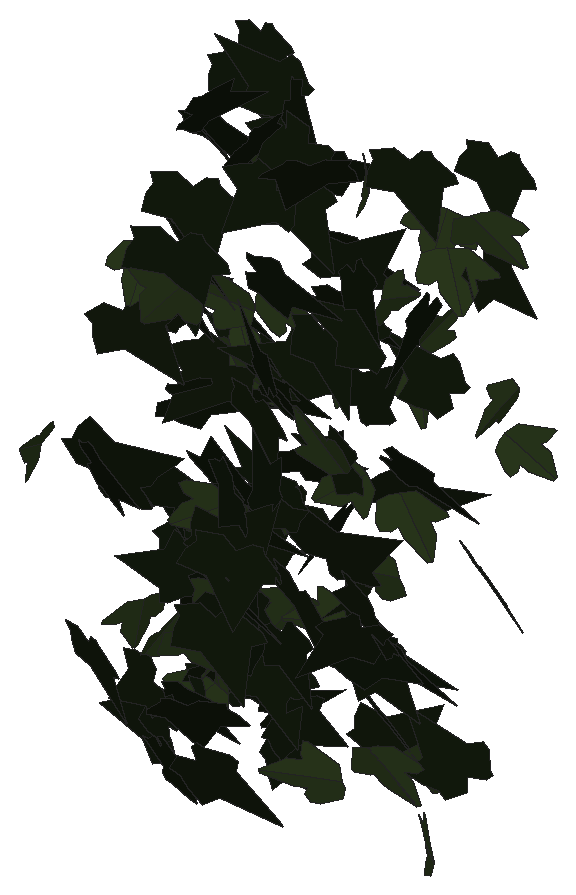
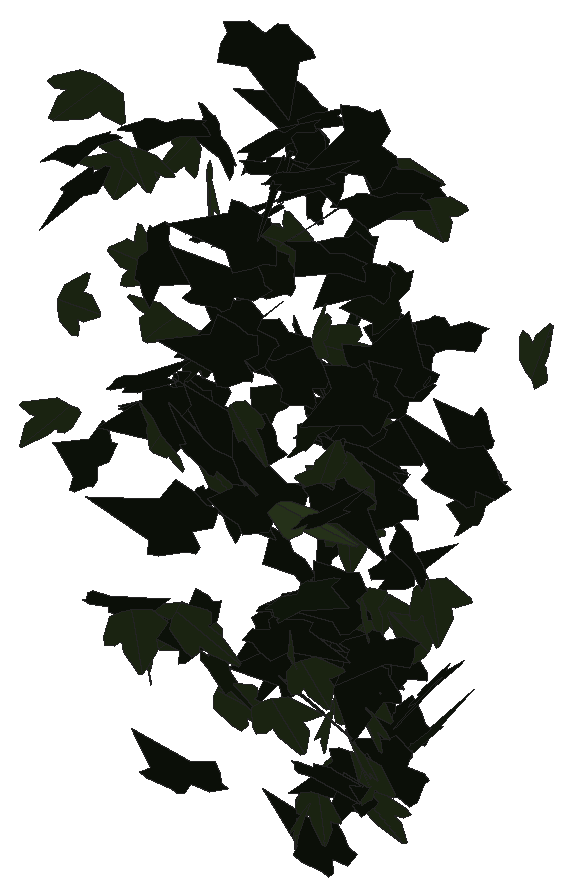
# SketchUp Ruby script. Lengths in inches.
U = 1.inch
M = Sketchup.active_model
def pt(a) = Geom::Point3d.new(a.map { |v| v * U })
def face(e, loops, mat)
  f = e.add_face(loops[0].map { |a| pt(a) })
  loops[1..].each { |l| e.add_face(l.map { |a| pt(a) }).erase! }
  f.material = f.back_material = mat if mat
  f
end
# faces: each face lists its corners as indices into pts; further lists are holes
def faces(e, pts, list, mat = nil) = list.each { |f| face(e, (f[0].is_a?(Array) ? f : [f]).map { |l| l.map { |i| pts[i] } }, mat) }
# xy, xz, yz: faces in a plane at the given z, y or x. An outline is a flat list of corners, or four numbers for a rectangle; further outlines are holes
def ring(l) = l.size == 4 ? [[l[0], l[1]], [l[2], l[1]], [l[2], l[3]], [l[0], l[3]]] : l.each_slice(2).to_a
def flat(e, list, mat, &to3) = list.each { |f| face(e, (f[0].is_a?(Array) ? f : [f]).map { |l| ring(l).map { |u, v| to3.(u, v) } }, mat) }
def xy(e, z, list, mat = nil) = flat(e, list, mat) { |x, y| [x, y, z] }
def xz(e, y, list, mat = nil) = flat(e, list, mat) { |x, z| [x, y, z] }
def yz(e, x, list, mat = nil) = flat(e, list, mat) { |y, z| [x, y, z] }
def lines(e, pts, list) = list.each { |a, b| e.add_line(pt(pts[a]), pt(pts[b])) }
# prism: a flat outline (further loops are holes) pulled along v
def prism(e, loops, v, mat = nil)
  f = face(e, loops, mat); d = Geom::Vector3d.new(v.map { |x| x * U })
  f.pushpull(f.normal.samedirection?(d) ? d.length : -d.length)
end
def box(e, o, s, mat = nil) = prism(e, [[o, [o[0] + s[0], o[1], o[2]], [o[0] + s[0], o[1] + s[1], o[2]], [o[0], o[1] + s[1], o[2]]]], [0, 0, s[2]], mat)
def at(x, y, z, deg = 0) = Geom::Transformation.translation(pt([x, y, z])) * Geom::Transformation.rotation(ORIGIN, Z_AXIS, deg.degrees)
def axes(o, x, y, z) = Geom::Transformation.new([*x, 0, *y, 0, *z, 0, *pt(o).to_a, 1])
def part(name) = M.definitions.add(name)
# library, detail: a bought-in or finely detailed component or shape, given as its bounding box
def library(name, o, s) = part(name).tap { |d| box(d.entities, o, s) }
def detail(e, o, s) = box(e.add_group.entities, o, s)
def put(e, d, t, mat = nil) = e.add_instance(d, t).tap { |i| i.material = mat if mat }
def group(e, t, mat = nil) = e.add_group.tap { |g| g.transformation = t; g.material = mat if mat }.entities
root = M.entities
M.materials.add("1026 AP 7946 SUNNY SIDE UP").color = [254, 231, 186]
M.materials.add("efeu1").color = [18, 25, 13]
M.materials.add("efeu2").color = [43, 57, 29]
c1 = part("ivyleaf_10")
p = [[0,0.5,-0.03],[-0.0625,2.02,-0.43],[-0.19,2.01,-0.46],[-0.54,1.05,-0.29],[-0.52,0.625,-0.18],[-0.83,0.76,-0.28],
  [-1.16,0.64,-0.33],[-1.15,0.33,-0.24],[-0.77,-0.39,0.02],[-0.3,-0.51,0.16],[0.04,-0.48,0.23],[-0.02,2.01,-0.4375],
  [-0.06,2.01,-0.43],[0.04,-0.49,0.23],[0.67,-0.49,0.14],[1.38,0.36,-0.2],[1.375,0.51,-0.24],[0.81,0.65,-0.19],
  [0.62,0.59,-0.15],[0.6,1.09,-0.28],[0.5,1.23,-0.31]]
faces(c1.entities,p,[[0,1,2,3,4,5,6,7,8,9,10],[11,12,0,13,14,15,16,17,18,19,20]],"efeu2")
c2 = part("ivyleaf_9")
p = [[1.54,2.16,1.25],[1.36,2.04,1.19],[-0.21,0.99,0.68],[-0.71,1.11,0.82],[-0.85,0.86,0.67],[-0.8,0.17,0.21],
  [-0.9,-0.01,0.1],[-0.67,-0.16,-0.02],[-0.08,-0.08,-0.05],[-0.03,-0.6,-0.4],[0.65,-0.88,-0.66],[0.83,-0.6,-0.49],
  [1.29,-0.42,-0.43],[1.8125,-0.07,-0.26],[1.21,0.44,0.15]]
faces(c2.entities,p,[[0,1,2,3,4,5,6,7,8,9,10,11,12,13,14]],"efeu1")
put(root,c1,axes([146.03,210.89,268.21],[0.51311,-0.04358,-0.15079],[-0.23302,-0.00932,-0.33813],[0.05649,0.35743,-0.02508]),"1026 AP 7946 SUNNY SIDE UP")
put(root,c1,axes([146.1,212.13,268.65],[-0.43066,0.1013,0.0913],[-0.15532,-0.01666,-0.29689],[-0.14289,-0.28721,0.04753]),"1026 AP 7946 SUNNY SIDE UP")
put(root,c2,axes([145.86,210.17,275.17],[-0.13859,-0.11339,0.38124],[0.43929,0.24499,0.14706],[-0.42261,0.29185,0.02784]),"1026 AP 7946 SUNNY SIDE UP")
put(root,c2,axes([146.11,212.16,269.29],[-0.46516,-0.0876,-0.02486],[0.04702,-0.01802,-0.31684],[0.13469,-0.29622,0.02473]),"1026 AP 7946 SUNNY SIDE UP")
put(root,c2,axes([146,210.41,275.59],[0.46379,0.03026,0.24064],[-0.36999,0.02876,0.30264],[0.00905,-0.37504,0.0404]),"1026 AP 7946 SUNNY SIDE UP")
put(root,c1,axes([145.95,206.91,274.29],[-0.06245,-0.16128,-0.37297],[-0.03983,-0.36115,0.16692],[-0.62061,0.03941,0.02682]),"1026 AP 7946 SUNNY SIDE UP")
put(root,c2,axes([145.77,211.24,278.11],[0.58075,0.02789,-0.01898],[-0.02481,-0.03668,-0.38005],[-0.04648,0.36799,-0.03426]),"1026 AP 7946 SUNNY SIDE UP")
put(root,c2,axes([145.84,210.78,271.06],[-0.03009,-0.20735,-0.30632],[0.04848,0.29456,-0.21278],[0.56641,-0.03623,0.00194]),"1026 AP 7946 SUNNY SIDE UP")
put(root,c2,axes([145.8,212.23,278.71],[-0.19436,-0.20395,-0.25893],[0.31752,0.16014,-0.23633],[0.39595,-0.22853,0.06242]),"1026 AP 7946 SUNNY SIDE UP")
put(root,c1,axes([146.18,212.29,271.09],[-0.25003,-0.23891,0.12707],[-0.08539,-0.11342,-0.29584],[0.41506,-0.16725,0.01568]),"1026 AP 7946 SUNNY SIDE UP")
put(root,c1,axes([146.04,211.91,270.16],[-0.12341,0.31857,-0.00557],[-0.05768,-0.01641,-0.33564],[-0.49772,-0.07709,0.04028]),"1026 AP 7946 SUNNY SIDE UP")
put(root,c1,axes([146.125,211.03,268.8125],[-0.56498,0.01557,-0.01993],[0.02818,-0.03347,-0.36917],[-0.02718,-0.35827,0.0315]),"1026 AP 7946 SUNNY SIDE UP")
put(root,c2,axes([146.32,212,273.59],[-0.21353,-0.32852,0.02303],[0.02423,0.01984,0.36627],[-0.51741,0.13651,0.00764]),"1026 AP 7946 SUNNY SIDE UP")
put(root,c2,axes([146.44,211.25,273.74],[0.13117,0.07271,-0.34449],[-0.47053,-0.15233,-0.11178],[-0.26233,0.30959,0.02825]),"1026 AP 7946 SUNNY SIDE UP")
put(root,c2,axes([146.18,211.16,268.12],[-0.28589,-0.15447,0.28414],[0.31328,0.19233,0.24662],[-0.38747,0.26948,-0.01025]),"1026 AP 7946 SUNNY SIDE UP")
put(root,c2,axes([145.86,210.05,272.39],[-0.09136,-0.06056,-0.35368],[0.54429,-0.04833,-0.05191],[-0.0603,-0.34448,0.06734]),"1026 AP 7946 SUNNY SIDE UP")
put(root,c1,axes([146.16,211.06,269.15],[0.39443,-0.25396,0.04214],[0.02631,-0.04292,-0.36751],[0.40398,0.25075,-0.01721]),"1026 AP 7946 SUNNY SIDE UP")
put(root,c2,axes([145.99,209.9,275.98],[0.62424,-0.05049,-0.10838],[-0.16712,-0.00495,-0.4119],[0.07474,0.41059,-0.01585]),"1026 AP 7946 SUNNY SIDE UP")
put(root,c2,axes([145.98,212.4,279.24],[0.11147,-0.33067,-0.0324],[0.01902,0.03279,-0.34767],[0.52167,0.06946,0.0196]),"1026 AP 7946 SUNNY SIDE UP")
put(root,c1,axes([146.2,210.86,269.76],[0.45748,-0.21713,0.01604],[-0.00333,-0.03086,-0.37321],[0.34241,0.28979,-0.02506]),"1026 AP 7946 SUNNY SIDE UP")
put(root,c2,axes([145.75,208.7,272.99],[-0.05988,0.05864,0.47119],[0.55918,-0.28789,0.06689],[0.46075,0.35702,-0.01995]),"1026 AP 7946 SUNNY SIDE UP")
put(root,c2,axes([146.27,210.82,270.4],[0.44196,0.1809,-0.16972],[-0.19488,-0.11288,-0.34405],[-0.33298,0.30617,-0.02391]),"1026 AP 7946 SUNNY SIDE UP")
put(root,c1,axes([146.22,210.7,271.51],[0.11166,-0.34717,0.13501],[0.10401,-0.12147,-0.36368],[0.57527,0.08935,0.03955]),"1026 AP 7946 SUNNY SIDE UP")
put(root,c2,axes([145.85,212.15,267.82],[0.04046,0.0225,0.39755],[0.41704,-0.28221,-0.00292],[0.4419,0.26427,-0.03364]),"1026 AP 7946 SUNNY SIDE UP")
put(root,c1,axes([146.12,212.08,277.04],[0.01319,-0.02855,0.36418],[0.26335,-0.31156,-0.03183],[0.49185,0.16758,0.00728]),"1026 AP 7946 SUNNY SIDE UP")
put(root,c2,axes([145.97,210.13,268.48],[0.56978,0.02817,0.06004],[0.09466,-0.02735,-0.37318],[-0.03678,0.36598,-0.03034]),"1026 AP 7946 SUNNY SIDE UP")
put(root,c2,axes([146.35,209.3,268.39],[0.16763,-0.3765,-0.12068],[0.07045,-0.10677,0.40225],[-0.61499,-0.11486,0.01319]),"1026 AP 7946 SUNNY SIDE UP")
put(root,c2,axes([146,210.45,270.17],[-0.01325,-0.03745,-0.39463],[0.57181,-0.12565,0.00368],[-0.19725,-0.36175,0.03718]),"1026 AP 7946 SUNNY SIDE UP")
put(root,c2,axes([145.95,210.39,273.61],[0.16332,0.18033,-0.33896],[0.17572,0.31214,0.21375],[0.56467,-0.14929,0.03152]),"1026 AP 7946 SUNNY SIDE UP")
put(root,c2,axes([146.11,210.9375,268.67],[0.01821,0.12631,-0.34181],[0.04095,0.33149,0.13259],[0.55779,-0.02846,0.00143]),"1026 AP 7946 SUNNY SIDE UP")
put(root,c2,axes([146.07,208.9,275.82],[-0.00536,-0.2593,-0.31849],[0.10384,0.30316,-0.26219],[0.62412,-0.05267,0.04088]),"1026 AP 7946 SUNNY SIDE UP")
put(root,c2,axes([146.38,209.13,269.25],[-0.15293,-0.13838,0.30876],[-0.18607,-0.27794,-0.17294],[0.48577,-0.15003,0.03096]),"1026 AP 7946 SUNNY SIDE UP")
put(root,c2,axes([146.62,212.07,270.53],[-0.4765,0.10981,-0.0185],[0.00923,-0.03805,-0.33045],[-0.17487,-0.30121,0.03298]),"1026 AP 7946 SUNNY SIDE UP")
put(root,c1,axes([146.29,210.875,270.07],[-0.54944,-0.02748,-0.10996],[0.17303,-0.09498,-0.34699],[-0.00379,-0.35276,0.09976]),"1026 AP 7946 SUNNY SIDE UP")
put(root,c2,axes([146.04,210.9,275.48],[0.58065,-0.02602,0.05002],[0.07125,-0.04539,-0.3792],[0.04961,0.3697,-0.04083]),"1026 AP 7946 SUNNY SIDE UP")
put(root,c2,axes([146.6,210.73,274.26],[-0.64525,-0.08014,-0.0421],[0.07483,-0.03393,-0.42873],[0.11965,-0.41095,0.0411]),"1026 AP 7946 SUNNY SIDE UP")
put(root,c1,axes([145.97,211.18,273.96],[0.02417,0.01341,0.38242],[0.58104,0.03648,-0.01691],[-0.05822,0.36966,-0.01002]),"1026 AP 7946 SUNNY SIDE UP")
put(root,c2,axes([145.96,208.24,273.37],[0.35547,-0.09435,-0.34014],[0.52022,-0.04364,0.24636],[-0.14155,-0.39732,0.05123]),"1026 AP 7946 SUNNY SIDE UP")
put(root,c1,axes([146.38,212.1,268.43],[-0.11609,0.30701,-0.02288],[-0.00028,-0.02467,-0.32538],[-0.4842,-0.07359,0.00567]),"1026 AP 7946 SUNNY SIDE UP")
put(root,c1,axes([146.5,208.74,270.81],[-0.18856,-0.38093,-0.01067],[0.02363,0.00386,-0.41117],[0.59865,-0.12014,0.01287]),"1026 AP 7946 SUNNY SIDE UP")
put(root,c1,axes([146.92,211.72,273.41],[-0.02114,0.39404,-0.0042],[-0.61943,-0.01326,0.01156],[0.01741,0.00669,0.40605]),"1026 AP 7946 SUNNY SIDE UP")
put(root,c1,axes([146.58,211.32,274.04],[0.23909,0.34678,-0.01481],[-0.01807,0.02286,0.38969],[0.54558,-0.15121,0.0194]),"1026 AP 7946 SUNNY SIDE UP")
put(root,c2,axes([146.17,210.09,276.8125],[0.40548,-0.30449,0.09589],[0.06483,-0.08907,-0.41075],[0.49724,0.25991,-0.02464]),"1026 AP 7946 SUNNY SIDE UP")
put(root,c2,axes([146.16,211.02,277.94],[0.33531,-0.24997,0.18097],[0.17062,-0.14014,-0.33923],[0.45046,0.23915,-0.00622]),"1026 AP 7946 SUNNY SIDE UP")
put(root,c2,axes([146.99,211.47,271.83],[-0.09134,0.37472,-0.03365],[-0.59151,-0.05683,0.01614],[0.01658,0.03681,0.39051]),"1026 AP 7946 SUNNY SIDE UP")
put(root,c2,axes([146.76,209.04,268.68],[-0.131,-0.28723,0.17665],[0.06697,0.16786,0.30903],[-0.52305,0.09343,-0.00467]),"1026 AP 7946 SUNNY SIDE UP")
put(root,c1,axes([146.81,211.66,268.11],[-0.09731,0.11465,0.31717],[-0.27974,0.25089,-0.13191],[-0.43313,-0.1878,0.01394]),"1026 AP 7946 SUNNY SIDE UP")
put(root,c1,axes([146.39,212.3125,271.1875],[0.16783,-0.07137,0.29712],[0.342,-0.19063,-0.13245],[0.31917,0.2418,-0.01431]),"1026 AP 7946 SUNNY SIDE UP")
put(root,c1,axes([146.57,209.01,270.01],[0.03545,-0.31474,0.17529],[0.01701,0.1728,0.32541],[-0.56368,-0.01458,0.02084]),"1026 AP 7946 SUNNY SIDE UP")
put(root,c2,axes([146.89,209.36,271.25],[-0.11728,-0.01335,0.37321],[-0.44759,-0.227,-0.0703],[0.35317,-0.29212,0.03483]),"1026 AP 7946 SUNNY SIDE UP")
put(root,c1,axes([147.125,210.33,275.73],[-0.0344,-0.00908,-0.39196],[-0.58945,0.06599,0.02097],[0.10282,0.3753,-0.0109]),"1026 AP 7946 SUNNY SIDE UP")
put(root,c2,axes([147.07,212.01,271.38],[-0.00307,-0.04884,-0.34484],[-0.20054,-0.30964,0.04554],[-0.4922,0.12646,-0.0164]),"1026 AP 7946 SUNNY SIDE UP")
put(root,c2,axes([146.75,209.79,279.25],[0.22959,0.20046,0.36382],[0.35365,0.2711,-0.25356],[-0.52978,0.26784,-0.01159]),"1026 AP 7946 SUNNY SIDE UP")
put(root,c2,axes([146.52,210.74,271.56],[0.46683,0.0114,0.20353],[0.30996,-0.04711,-0.30274],[0.02625,0.35345,-0.04481]),"1026 AP 7946 SUNNY SIDE UP")
put(root,c1,axes([146.95,208.28,277.42],[0.44226,0.23963,-0.11085],[-0.09922,-0.09343,-0.38003],[-0.40186,0.28679,-0.02816]),"1026 AP 7946 SUNNY SIDE UP")
put(root,c1,axes([147.18,211.78,269.8],[-0.38871,-0.17507,0.15817],[-0.16648,-0.11654,-0.3112],[0.32727,-0.26722,0.02956]),"1026 AP 7946 SUNNY SIDE UP")
put(root,c2,axes([147.3125,211.4,279.09],[-0.33987,-0.30657,-0.04865],[-0.06146,-0.02804,0.38593],[-0.48344,0.21909,-0.01487]),"1026 AP 7946 SUNNY SIDE UP")
put(root,c2,axes([146.95,209.47,278.08],[-0.20158,-0.35924,-0.16119],[0.13981,0.13147,-0.39036],[0.59874,-0.15165,0.03688]),"1026 AP 7946 SUNNY SIDE UP")
put(root,c1,axes([147.3,209.85,272.26],[-0.20481,-0.34476,-0.03407],[0.03835,0.02402,-0.37925],[0.54295,-0.13174,0.01393]),"1026 AP 7946 SUNNY SIDE UP")
put(root,c2,axes([146.92,208.83,268.07],[0.13754,-0.10289,0.36132],[0.34114,-0.27636,-0.14065],[0.46363,0.23387,-0.0037]),"1026 AP 7946 SUNNY SIDE UP")
put(root,c1,axes([147.3125,209,270.43],[-0.42794,-0.1874,-0.19156],[0.26256,0.08268,-0.33909],[0.32,-0.31845,0.02205]),"1026 AP 7946 SUNNY SIDE UP")
put(root,c2,axes([147.14,206.66,271.25],[0.23797,-0.35954,0.13376],[0.05757,-0.12758,-0.40232],[0.59942,0.15499,-0.01447]),"1026 AP 7946 SUNNY SIDE UP")
put(root,c2,axes([147.55,208.63,269.42],[0.40997,0.26246,-0.12501],[-0.11612,-0.0996,-0.38131],[-0.44062,0.27046,-0.01582]),"1026 AP 7946 SUNNY SIDE UP")
put(root,c2,axes([147.61,210.07,278.91],[-0.11824,0.10912,-0.40439],[-0.25538,0.35873,0.13668],[0.58855,0.17759,-0.02194]),"1026 AP 7946 SUNNY SIDE UP")
put(root,c2,axes([147.6,211.13,279.16],[0.22441,-0.17512,-0.35127],[-0.40147,0.22654,-0.2293],[0.44769,0.29092,-0.02955]),"1026 AP 7946 SUNNY SIDE UP")
put(root,c2,axes([147.17,210.04,270.57],[0.01318,-0.11884,-0.37982],[0.52152,0.19151,-0.05481],[0.31272,-0.31437,0.10741]),"1026 AP 7946 SUNNY SIDE UP")
put(root,c1,axes([148.06,211.84,269.72],[-0.16656,0.02336,0.35767],[-0.50159,-0.15117,-0.09071],[0.21806,-0.32987,0.06455]),"1026 AP 7946 SUNNY SIDE UP")
put(root,c2,axes([147.28,208.69,272.89],[0.01134,0.00151,0.41503],[0.63219,0.02536,-0.00737],[-0.03991,0.40212,0.00127]),"1026 AP 7946 SUNNY SIDE UP")
put(root,c1,axes([148,207.68,277.39],[-0.51814,-0.03369,0.21366],[-0.31003,-0.08474,-0.3371],[0.11504,-0.38013,0.05386]),"1026 AP 7946 SUNNY SIDE UP")
put(root,c2,axes([147.51,210.36,274.05],[0.09951,-0.35126,0.16048],[0.05369,-0.15414,-0.36855],[0.6031,0.07168,0.00633]),"1026 AP 7946 SUNNY SIDE UP")
put(root,c2,axes([147.58,208.27,277.83],[-0.39104,-0.2164,-0.29725],[0.39045,0.1494,-0.33648],[0.40916,-0.34939,0.03702]),"1026 AP 7946 SUNNY SIDE UP")
put(root,c2,axes([148.2,210.7,278.8125],[-0.50601,-0.18464,0.06519],[-0.06264,-0.05938,-0.38121],[0.30099,-0.32276,0.03027]),"1026 AP 7946 SUNNY SIDE UP")
put(root,c2,axes([147.99,209.09,273.32],[0.52417,-0.1888,0.14838],[-0.16778,0.10473,0.39354],[-0.33472,-0.34816,0.0351]),"1026 AP 7946 SUNNY SIDE UP")
put(root,c1,axes([148.28,211.32,274.51],[0.28395,-0.12768,-0.30903],[-0.29916,0.23619,-0.22071],[0.41499,0.25763,0.05234]),"1026 AP 7946 SUNNY SIDE UP")
put(root,c2,axes([148.33,211.97,270.39],[-0.40943,0.22923,-0.10477],[0.0881,-0.09164,-0.35654],[-0.38522,-0.2646,0.02982]),"1026 AP 7946 SUNNY SIDE UP")
put(root,c2,axes([147.65,212.14,276.125],[0.38412,-0.08059,0.26078],[0.36018,-0.11149,-0.26447],[0.21291,0.334,-0.02308]),"1026 AP 7946 SUNNY SIDE UP")
put(root,c1,axes([148.41,208.25,273.48],[0.43206,-0.13412,-0.25309],[-0.38299,0.0529,-0.31106],[0.21471,0.36426,-0.04555]),"1026 AP 7946 SUNNY SIDE UP")
put(root,c2,axes([147.91,211,272.77],[0.55385,0.20066,0.08932],[-0.14445,-0.01096,0.41598],[0.31111,-0.36231,0.03412]),"1026 AP 7946 SUNNY SIDE UP")
put(root,c2,axes([147.91,211.39,277.93],[0.17545,0.1978,-0.2918],[0.15196,0.26912,0.23348],[0.52305,-0.14453,0.03005]),"1026 AP 7946 SUNNY SIDE UP")
put(root,c2,axes([147.87,210.12,274.6875],[0.22544,-0.10535,0.33726],[0.33907,-0.24959,-0.18117],[0.42241,0.25657,-0.03458]),"1026 AP 7946 SUNNY SIDE UP")
put(root,c2,axes([148.9,210.25,275.22],[-0.34962,0.00903,0.34817],[-0.52824,-0.0508,-0.22663],[0.059,-0.4013,0.03413]),"1026 AP 7946 SUNNY SIDE UP")
put(root,c1,axes([148.89,211.9,270.83],[-0.19052,0.02862,0.37021],[-0.5659,-0.02839,-0.1229],[0.02807,-0.37802,0.03502]),"1026 AP 7946 SUNNY SIDE UP")
put(root,c2,axes([148.6,208.64,270.7],[-0.13551,-0.14819,0.43001],[0.28478,0.37721,0.17833],[-0.63694,0.20018,-0.01175]),"1026 AP 7946 SUNNY SIDE UP")
put(root,c2,axes([148.7,209.29,278.76],[-0.32851,-0.24529,0.1872],[-0.1371,-0.16481,-0.33091],[0.46136,-0.22363,0.03495]),"1026 AP 7946 SUNNY SIDE UP")
put(root,c2,axes([148.14,208.16,268.83],[0.07186,-0.00795,-0.41111],[0.54714,0.19747,0.03816],[0.3073,-0.34972,0.02819]),"1026 AP 7946 SUNNY SIDE UP")
put(root,c2,axes([148.4,211.8125,273.76],[-0.23265,0.17991,0.28695],[0.29873,-0.20262,0.23849],[0.42568,0.24052,-0.01053]),"1026 AP 7946 SUNNY SIDE UP")
put(root,c2,axes([148.28,211.02,275.93],[0.56663,0.0495,0.11263],[0.17865,-0.03199,-0.37201],[-0.05953,0.37514,-0.04434]),"1026 AP 7946 SUNNY SIDE UP")
put(root,c2,axes([148.44,209.62,269.23],[0.14072,0.12046,0.35133],[0.41982,0.21396,-0.14909],[-0.38214,0.27941,-0.03441]),"1026 AP 7946 SUNNY SIDE UP")
put(root,c1,axes([148.97,210.95,272.99],[0.45351,-0.15078,-0.20749],[-0.30895,0.05431,-0.33284],[0.24537,0.34707,-0.0356]),"1026 AP 7946 SUNNY SIDE UP")
put(root,c2,axes([148.66,209.29,270.26],[-0.07178,-0.37873,-0.15914],[0.04124,0.15024,-0.39203],[0.64055,-0.05211,0.0074]),"1026 AP 7946 SUNNY SIDE UP")
put(root,c2,axes([148.65,211.09,276.48],[-0.1878,-0.02226,0.37125],[0.56002,0.05584,0.12544],[-0.09439,0.37563,0.00561]),"1026 AP 7946 SUNNY SIDE UP")
put(root,c2,axes([149.01,210.62,272.52],[-0.24553,0.15333,-0.31696],[0.26991,-0.2591,-0.22365],[-0.46974,-0.22902,0.03717]),"1026 AP 7946 SUNNY SIDE UP")
put(root,c1,axes([148.49,209.49,276.65],[0.10292,0.00221,0.39294],[0.59949,0.01076,-0.0674],[-0.01726,0.38683,0.00189]),"1026 AP 7946 SUNNY SIDE UP")
put(root,c2,axes([148.51,207.77,272.66],[0.55511,-0.21894,0.12725],[0.137,-0.09545,-0.42711],[0.37181,0.36206,-0.03261]),"1026 AP 7946 SUNNY SIDE UP")
put(root,c2,axes([148.79,209.63,278.68],[0.07265,-0.38059,-0.19263],[-0.00267,0.18576,-0.3934],[0.66527,0.04231,0.01946]),"1026 AP 7946 SUNNY SIDE UP")
put(root,c1,axes([149.19,210.96,278.27],[0.03056,-0.1205,-0.36845],[-0.13151,0.34715,-0.12338],[0.57764,0.08541,-0.0086]),"1026 AP 7946 SUNNY SIDE UP")
put(root,c2,axes([149.32,208.33,273.88],[0.00424,0.08177,0.42131],[-0.09616,0.40416,-0.08056],[-0.64797,-0.05945,0.01471]),"1026 AP 7946 SUNNY SIDE UP")
put(root,c2,axes([148.94,207.99,274.02],[-0.03484,-0.19801,0.36149],[-0.06182,-0.34982,-0.2073],[0.63206,-0.04513,-0.00035]),"1026 AP 7946 SUNNY SIDE UP")
put(root,c2,axes([148.97,209.2,269.05],[0.18081,-0.23947,-0.31488],[-0.21717,0.27118,-0.27204],[0.56881,0.17966,-0.00377]),"1026 AP 7946 SUNNY SIDE UP")
put(root,c2,axes([148.92,207.6,271.9],[-0.10267,-0.38422,-0.1568],[0.09267,0.14164,-0.3993],[0.64191,-0.0819,0.03257]),"1026 AP 7946 SUNNY SIDE UP")
put(root,c2,axes([148.96,207.78,273],[-0.3641,0.15555,0.3024],[0.42383,-0.11934,0.28436],[0.30322,0.35359,-0.03435]),"1026 AP 7946 SUNNY SIDE UP")
put(root,c2,axes([148.9375,209.23,270.92],[-0.1798,-0.05703,-0.34771],[0.53377,0.02421,-0.12267],[0.06525,-0.35523,0.04532]),"1026 AP 7946 SUNNY SIDE UP")
put(root,c2,axes([149.12,209.15,269.55],[0.0614,-0.0521,-0.38326],[-0.13724,0.36223,-0.05963],[0.57405,0.09217,0.02674]),"1026 AP 7946 SUNNY SIDE UP")
put(root,c2,axes([149.01,211.73,267.86],[-0.27365,0.07415,0.31953],[0.48091,-0.05958,0.19138],[0.13974,0.35026,-0.03289]),"1026 AP 7946 SUNNY SIDE UP")
put(root,c1,axes([149.04,212.36,274.31],[0.42494,-0.1088,0.28192],[0.36569,-0.15034,-0.2984],[0.28552,0.35448,-0.03739]),"1026 AP 7946 SUNNY SIDE UP")
put(root,c2,axes([149.35,207.52,273.29],[-0.36663,-0.28075,-0.14888],[0.17785,0.09135,-0.37443],[0.46234,-0.25778,0.02597]),"1026 AP 7946 SUNNY SIDE UP")
put(root,c2,axes([149.76,207.78,276.42],[0.04164,-0.15607,0.36994],[-0.09972,0.35435,0.16515],[-0.60883,-0.06872,-0.00175]),"1026 AP 7946 SUNNY SIDE UP")
put(root,c2,axes([149.12,211.61,272.31],[0.16274,0.03796,0.41997],[0.63522,0.05752,-0.1109],[-0.10258,0.41643,-0.02046]),"1026 AP 7946 SUNNY SIDE UP")
put(root,c2,axes([149.76,208.86,279.74],[0.17099,0.34343,-0.19759],[-0.08376,-0.18634,-0.37217],[-0.61433,0.121,-0.00426]),"1026 AP 7946 SUNNY SIDE UP")
put(root,c2,axes([150.14,211.78,274.62],[-0.32336,-0.30432,-0.00107],[-0.01556,0.00752,0.37821],[-0.47826,0.20551,-0.01158]),"1026 AP 7946 SUNNY SIDE UP")
put(root,c2,axes([149.44,208.625,275.53],[0.28603,-0.25301,0.27467],[0.25742,-0.21236,-0.32219],[0.51928,0.24463,0.00843]),"1026 AP 7946 SUNNY SIDE UP")
put(root,c2,axes([149.38,208.14,278.01],[0.2916,0.00549,-0.35989],[0.527,0.10907,0.18567],[0.15539,-0.38021,0.04566]),"1026 AP 7946 SUNNY SIDE UP")
put(root,c2,axes([149.74,209.26,276.59],[0.06049,-0.41397,-0.04274],[-0.01161,0.03861,-0.42806],[0.65373,0.03899,-0.00365]),"1026 AP 7946 SUNNY SIDE UP")
put(root,c2,axes([150.09,209.42,274.31],[0.06582,-0.34818,-0.06966],[0.02037,-0.06454,0.36086],[-0.55676,-0.04352,0.00497]),"1026 AP 7946 SUNNY SIDE UP")
put(root,c2,axes([150.3,209.75,276.46],[-0.18982,-0.34969,-0.10054],[-0.02435,-0.09571,0.38019],[-0.56951,0.12065,0.01725]),"1026 AP 7946 SUNNY SIDE UP")
put(root,c2,axes([149.72,209.41,272.52],[-0.103,-0.0153,0.42596],[0.57202,-0.20176,0.05049],[0.31025,0.36691,0.04832]),"1026 AP 7946 SUNNY SIDE UP")
put(root,c2,axes([150.08,210.97,278.99],[-0.14768,-0.32893,-0.17247],[0.14812,0.14371,-0.34835],[0.55975,-0.12481,0.04668]),"1026 AP 7946 SUNNY SIDE UP")
put(root,c2,axes([149.91,210.25,269.63],[0.40971,-0.29482,0.12839],[0.09998,-0.11201,-0.40516],[0.49431,0.26702,-0.02447]),"1026 AP 7946 SUNNY SIDE UP")
put(root,c2,axes([149.98,210.8,273.68],[0.54735,-0.09869,0.13364],[0.18365,-0.06422,-0.37198],[0.17977,0.36609,-0.02687]),"1026 AP 7946 SUNNY SIDE UP")
put(root,c2,axes([150.13,208.15,272.57],[0.14131,-0.36246,0.26012],[0.08708,-0.24851,-0.38613],[0.69097,0.10544,-0.00453]),"1026 AP 7946 SUNNY SIDE UP")
put(root,c2,axes([150.44,210.91,276.52],[-0.17222,0.08801,-0.44491],[0.42698,-0.33769,-0.14365],[-0.54685,-0.29139,0.02795]),"1026 AP 7946 SUNNY SIDE UP")
put(root,c1,axes([150.83,208.08,275.24],[-0.45018,0.12899,-0.25263],[-0.35054,0.10392,0.32409],[0.26043,0.36285,-0.00045]),"1026 AP 7946 SUNNY SIDE UP")
put(root,c2,axes([150.41,209.2,277.875],[-0.1135,-0.04463,-0.37268],[0.56997,-0.04502,-0.0691],[-0.05629,-0.36588,0.05176]),"1026 AP 7946 SUNNY SIDE UP")
put(root,c1,axes([150.68,210.78,276.2],[0.08961,-0.24132,0.30276],[-0.03917,0.29555,0.25553],[-0.59833,-0.05549,0.02862]),"1026 AP 7946 SUNNY SIDE UP")
put(root,c1,axes([150.71,210.95,278.22],[0.5835,-0.00713,-0.00371],[-0.00664,-0.0353,-0.38083],[0.01063,0.36942,-0.03428]),"1026 AP 7946 SUNNY SIDE UP")
put(root,c1,axes([150.625,209.53,269.2],[-0.50638,-0.01633,-0.20349],[0.31149,-0.03085,-0.33043],[-0.00356,-0.37648,0.03368]),"1026 AP 7946 SUNNY SIDE UP")
put(root,c2,axes([150.79,209.13,271.29],[0.19437,-0.29004,-0.2835],[-0.15901,0.25422,-0.32327],[0.60639,0.15963,0.0061]),"1026 AP 7946 SUNNY SIDE UP")
put(root,c1,axes([150.92,209.35,277.625],[-0.06419,-0.13048,-0.34529],[0.1572,0.31913,-0.13897],[0.54213,-0.10799,-0.00059]),"1026 AP 7946 SUNNY SIDE UP")
put(root,c1,axes([151.42,207.2,270.14],[-0.11647,0.02384,0.3864],[-0.52834,-0.17516,-0.05794],[0.26426,-0.33968,0.05447]),"1026 AP 7946 SUNNY SIDE UP")
put(root,c2,axes([150.91,212.125,278.83],[-0.11211,-0.36428,-0.02369],[0.0139,0.01959,-0.38225],[0.57357,-0.07168,0.00463]),"1026 AP 7946 SUNNY SIDE UP")
put(root,c1,axes([151.3,210.23,269.24],[-0.36577,-0.3038,0.03044],[-0.00088,-0.03889,-0.39369],[0.48022,-0.23146,0.02247]),"1026 AP 7946 SUNNY SIDE UP")
put(root,c1,axes([151.14,210.64,277.75],[0.46949,0.23926,0.06176],[0.10424,0.01062,-0.39266],[-0.37304,0.30409,-0.03199]),"1026 AP 7946 SUNNY SIDE UP")
put(root,c1,axes([151.27,212.14,273.9],[0.1758,0.26606,0.24439],[0.12601,0.22187,-0.29586],[-0.54454,0.13724,0.01043]),"1026 AP 7946 SUNNY SIDE UP")
put(root,c2,axes([151.96,209.96,269.2],[-0.52061,-0.15899,-0.05455],[-0.09562,0.00688,0.37696],[-0.24506,0.33508,-0.03121]),"1026 AP 7946 SUNNY SIDE UP")
put(root,c2,axes([151.48,211.1,277.62],[0.1922,-0.20498,-0.31051],[-0.1668,0.28287,-0.24178],[0.54676,0.15835,0.03539]),"1026 AP 7946 SUNNY SIDE UP")
put(root,c1,axes([151.93,209.11,268.16],[-0.01134,0.04667,-0.4054],[-0.18421,0.37602,0.05032],[0.59569,0.11717,0.00784]),"1026 AP 7946 SUNNY SIDE UP")
put(root,c2,axes([151.71,208.01,272.77],[0.35023,-0.38956,-0.09196],[0.10712,-0.06112,0.46102],[-0.61845,-0.2312,0.02778]),"1026 AP 7946 SUNNY SIDE UP")
put(root,c1,axes([151.45,209.11,274.16],[0.49621,0.06997,0.21367],[0.32945,0.00636,-0.33122],[-0.09756,0.37736,-0.03176]),"1026 AP 7946 SUNNY SIDE UP")
put(root,c1,axes([151.78,211.27,275.3],[0.0322,-0.19936,0.33318],[0.08317,-0.32038,-0.20805],[0.59311,0.05575,0.01109]),"1026 AP 7946 SUNNY SIDE UP")
put(root,c2,axes([151.99,207.3,272.95],[-0.03307,0.12136,-0.37449],[0.02978,-0.36397,-0.12821],[-0.60289,-0.02463,0.01421]),"1026 AP 7946 SUNNY SIDE UP")
put(root,c2,axes([151.42,207.93,272.1],[0.11832,0.0795,-0.40905],[0.34773,0.33079,0.11322],[0.53422,-0.23293,0.0169]),"1026 AP 7946 SUNNY SIDE UP")
put(root,c2,axes([151.55,210.89,272.3],[0.2433,-0.27573,0.23762],[0.14715,-0.21333,-0.32642],[0.5474,0.17989,-0.01787]),"1026 AP 7946 SUNNY SIDE UP")
put(root,c2,axes([151.59,208.32,272.02],[0.43604,-0.1492,0.21171],[0.26376,-0.1225,-0.3242],[0.30124,0.32322,-0.02258]),"1026 AP 7946 SUNNY SIDE UP")
put(root,c1,axes([151.91,210.48,278.76],[-0.46583,-0.12389,-0.22482],[0.34407,0.03557,-0.32766],[0.19122,-0.36581,0.04187]),"1026 AP 7946 SUNNY SIDE UP")
